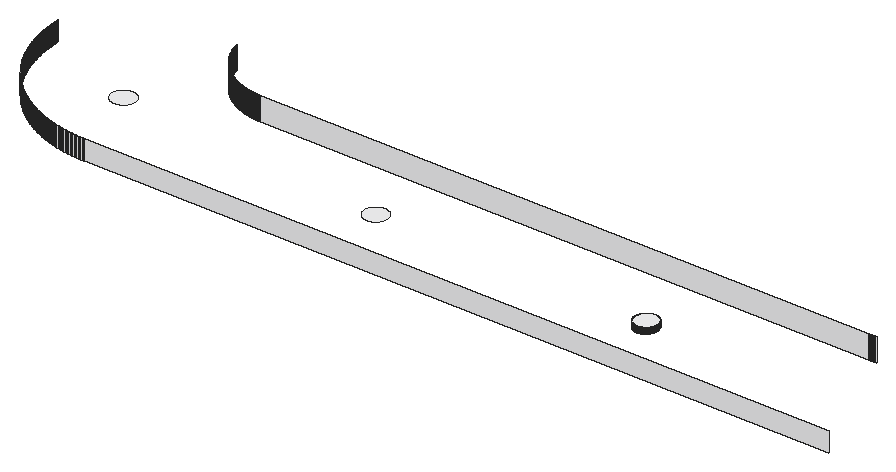
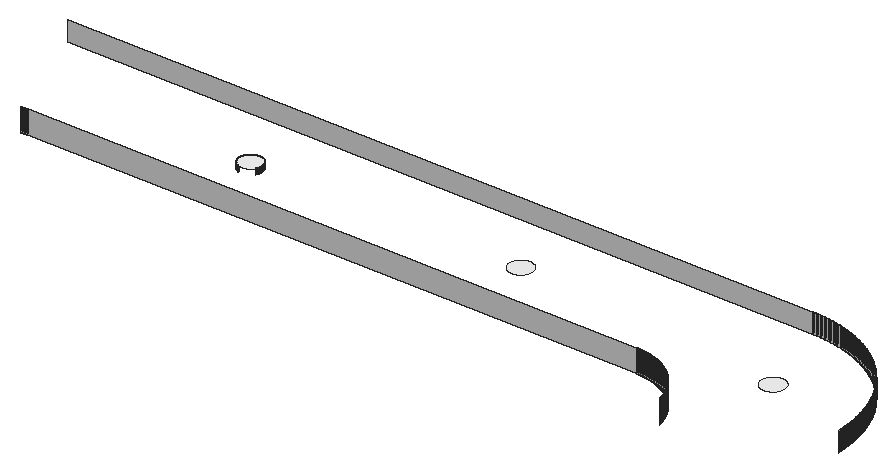
# SketchUp Ruby script. Lengths in inches.
U = 1.inch
M = Sketchup.active_model
def pt(a) = Geom::Point3d.new(a.map { |v| v * U })
def face(e, loops, mat)
  f = e.add_face(loops[0].map { |a| pt(a) })
  loops[1..].each { |l| e.add_face(l.map { |a| pt(a) }).erase! }
  f.material = f.back_material = mat if mat
  f
end
# faces: each face lists its corners as indices into pts; further lists are holes
def faces(e, pts, list, mat = nil) = list.each { |f| face(e, (f[0].is_a?(Array) ? f : [f]).map { |l| l.map { |i| pts[i] } }, mat) }
# xy, xz, yz: faces in a plane at the given z, y or x. An outline is a flat list of corners, or four numbers for a rectangle; further outlines are holes
def ring(l) = l.size == 4 ? [[l[0], l[1]], [l[2], l[1]], [l[2], l[3]], [l[0], l[3]]] : l.each_slice(2).to_a
def flat(e, list, mat, &to3) = list.each { |f| face(e, (f[0].is_a?(Array) ? f : [f]).map { |l| ring(l).map { |u, v| to3.(u, v) } }, mat) }
def xy(e, z, list, mat = nil) = flat(e, list, mat) { |x, y| [x, y, z] }
def xz(e, y, list, mat = nil) = flat(e, list, mat) { |x, z| [x, y, z] }
def yz(e, x, list, mat = nil) = flat(e, list, mat) { |y, z| [x, y, z] }
def lines(e, pts, list) = list.each { |a, b| e.add_line(pt(pts[a]), pt(pts[b])) }
# prism: a flat outline (further loops are holes) pulled along v
def prism(e, loops, v, mat = nil)
  f = face(e, loops, mat); d = Geom::Vector3d.new(v.map { |x| x * U })
  f.pushpull(f.normal.samedirection?(d) ? d.length : -d.length)
end
def box(e, o, s, mat = nil) = prism(e, [[o, [o[0] + s[0], o[1], o[2]], [o[0] + s[0], o[1] + s[1], o[2]], [o[0], o[1] + s[1], o[2]]]], [0, 0, s[2]], mat)
def at(x, y, z, deg = 0) = Geom::Transformation.translation(pt([x, y, z])) * Geom::Transformation.rotation(ORIGIN, Z_AXIS, deg.degrees)
def axes(o, x, y, z) = Geom::Transformation.new([*x, 0, *y, 0, *z, 0, *pt(o).to_a, 1])
def part(name) = M.definitions.add(name)
# library, detail: a bought-in or finely detailed component or shape, given as its bounding box
def library(name, o, s) = part(name).tap { |d| box(d.entities, o, s) }
def detail(e, o, s) = box(e.add_group.entities, o, s)
def put(e, d, t, mat = nil) = e.add_instance(d, t).tap { |i| i.material = mat if mat }
def group(e, t, mat = nil) = e.add_group.tap { |g| g.transformation = t; g.material = mat if mat }.entities
root = M.entities
M.materials.add("[Quartz Light Grey]").color = [251, 251, 252]
xy(root,112.81,[[87.021,52,86.896,52.003,86.771,52.013,86.646,52.032,86.523,52.058,86.402,52.091,86.284,52.133,86.168,52.181,86.055,52.237,85.947,52.3,85.842,52.369,85.742,52.445,85.647,52.527,85.557,52.615,85.473,52.709,85.395,52.807,85.323,52.91,85.258,53.018,85.2,53.129,85.148,53.244,85.105,53.362,85.068,53.482,85.04,53.604,85.019,53.728,85.005,53.853,85,53.979,85.003,54.104,85.013,54.229,85.032,54.354,85.058,54.477,85.091,54.598,85.133,54.716,85.181,54.832,85.237,54.945,85.3,55.053,85.369,55.158,85.445,55.258,85.527,55.353,85.615,55.443,85.709,55.527,85.807,55.605,85.91,55.677,86.018,55.742,86.129,55.8,86.244,55.852,86.362,55.895,86.482,55.932,86.604,55.96,86.728,55.981,86.853,55.995,86.979,56,87.104,55.997,87.229,55.987,87.354,55.968,87.477,55.942,87.598,55.909,87.716,55.867,87.832,55.819,87.945,55.763,88.053,55.7,88.158,55.631,88.258,55.555,88.353,55.473,88.443,55.385,88.527,55.291,88.605,55.193,88.677,55.09,88.742,54.982,88.8,54.871,88.852,54.756,88.895,54.638,88.932,54.518,88.96,54.396,88.981,54.272,88.995,54.147,89,54.021,88.997,53.896,88.987,53.771,88.968,53.646,88.942,53.523,88.909,53.402,88.867,53.284,88.819,53.168,88.763,53.055,88.7,52.947,88.631,52.842,88.555,52.742,88.473,52.647,88.385,52.557,88.291,52.473,88.193,52.395,88.09,52.323,87.982,52.258,87.871,52.2,87.756,52.148,87.638,52.105,87.518,52.068,87.396,52.04,87.272,52.019,87.147,52.005],[135.021,52,134.896,52.003,134.771,52.013,134.646,52.032,134.523,52.058,134.402,52.091,134.284,52.133,134.168,52.181,134.055,52.237,133.947,52.3,133.842,52.369,133.742,52.445,133.647,52.527,133.557,52.615,133.473,52.709,133.395,52.807,133.323,52.91,133.258,53.018,133.2,53.129,133.148,53.244,133.105,53.362,133.068,53.482,133.04,53.604,133.019,53.728,133.005,53.853,133,53.979,133.003,54.104,133.013,54.229,133.032,54.354,133.058,54.477,133.091,54.598,133.133,54.716,133.181,54.832,133.237,54.945,133.3,55.053,133.369,55.158,133.445,55.258,133.527,55.353,133.615,55.443,133.709,55.527,133.807,55.605,133.91,55.677,134.018,55.742,134.129,55.8,134.244,55.852,134.362,55.895,134.482,55.932,134.604,55.96,134.728,55.981,134.853,55.995,134.979,56,135.104,55.997,135.229,55.987,135.354,55.968,135.477,55.942,135.598,55.909,135.716,55.867,135.832,55.819,135.945,55.763,136.053,55.7,136.158,55.631,136.258,55.555,136.353,55.473,136.443,55.385,136.527,55.291,136.605,55.193,136.677,55.09,136.742,54.982,136.8,54.871,136.852,54.756,136.895,54.638,136.932,54.518,136.96,54.396,136.981,54.272,136.995,54.147,137,54.021,136.997,53.896,136.987,53.771,136.968,53.646,136.942,53.523,136.909,53.402,136.867,53.284,136.819,53.168,136.763,53.055,136.7,52.947,136.631,52.842,136.555,52.742,136.473,52.647,136.385,52.557,136.291,52.473,136.193,52.395,136.09,52.323,135.982,52.258,135.871,52.2,135.756,52.148,135.638,52.105,135.518,52.068,135.396,52.04,135.272,52.019,135.147,52.005],[39.021,56,38.896,56.003,38.771,56.013,38.646,56.032,38.523,56.058,38.402,56.091,38.284,56.133,38.168,56.181,38.055,56.237,37.947,56.3,37.842,56.369,37.742,56.445,37.647,56.527,37.557,56.615,37.473,56.709,37.395,56.807,37.323,56.91,37.258,57.018,37.2,57.129,37.148,57.244,37.105,57.362,37.068,57.482,37.04,57.604,37.019,57.728,37.005,57.853,37,57.979,37.003,58.104,37.013,58.229,37.032,58.354,37.058,58.477,37.091,58.598,37.133,58.716,37.181,58.832,37.237,58.945,37.3,59.053,37.369,59.158,37.445,59.258,37.527,59.353,37.615,59.443,37.709,59.527,37.807,59.605,37.91,59.677,38.018,59.742,38.129,59.8,38.244,59.852,38.362,59.895,38.482,59.932,38.604,59.96,38.728,59.981,38.853,59.995,38.979,60,39.104,59.997,39.229,59.987,39.354,59.968,39.477,59.942,39.598,59.909,39.716,59.867,39.832,59.819,39.945,59.763,40.053,59.7,40.158,59.631,40.258,59.555,40.353,59.473,40.443,59.385,40.527,59.291,40.605,59.193,40.677,59.09,40.742,58.982,40.8,58.871,40.852,58.756,40.895,58.638,40.932,58.518,40.96,58.396,40.981,58.272,40.995,58.147,41,58.021,40.997,57.896,40.987,57.771,40.968,57.646,40.942,57.523,40.909,57.402,40.867,57.284,40.819,57.168,40.763,57.055,40.7,56.947,40.631,56.842,40.555,56.742,40.473,56.647,40.385,56.557,40.291,56.473,40.193,56.395,40.09,56.323,39.982,56.258,39.871,56.2,39.756,56.148,39.638,56.105,39.518,56.068,39.396,56.04,39.272,56.019,39.147,56.005]],"[Quartz Light Grey]")
xz(root,42,[[45,111.81,177,115.32]],"[Quartz Light Grey]")
xz(root,66,[[57,111.81,165,115.905]],"[Quartz Light Grey]")
p = [[43.242,42.064,111.81],[43.493,42.047,111.81],[43.493,42.047,115.32],[43.242,42.064,115.32],[43.744,42.033,111.81],[43.744,42.033,115.32],
  [43.995,42.021,111.81],[43.995,42.021,115.32],[44.246,42.012,111.81],[44.246,42.012,115.32],[44.497,42.005,111.81],[44.497,42.005,115.32],
  [44.749,42.001,111.81],[44.749,42.001,115.32],[45,42,111.81],[45,42,115.32],[42.242,42.159,111.81],[42.491,42.131,111.81],
  [42.491,42.131,115.32],[42.242,42.159,115.32],[42.741,42.107,111.81],[42.741,42.107,115.32],[42.992,42.084,111.81],[42.992,42.084,115.32],
  [41.494,42.257,111.81],[41.743,42.222,111.81],[41.743,42.222,115.32],[41.494,42.257,115.32],[41.992,42.189,111.81],[41.992,42.189,115.32],
  [40.75,42.379,111.81],[40.998,42.336,111.81],[40.998,42.336,115.32],[40.75,42.379,115.32],[41.246,42.295,111.81],[41.246,42.295,115.32],
  [40.256,42.473,111.81],[40.503,42.425,111.81],[40.503,42.425,115.32],[40.256,42.473,115.32],[39.765,42.578,111.81],[40.01,42.524,111.81],
  [40.01,42.524,115.32],[39.765,42.578,115.32],[39.275,42.693,111.81],[39.52,42.634,111.81],[39.52,42.634,115.32],[39.275,42.693,115.32],
  [39.031,42.754,111.81],[39.031,42.754,115.32],[38.546,42.884,111.81],[38.788,42.818,111.81],[38.788,42.818,115.32],[38.546,42.884,115.32],
  [38.304,42.953,111.81],[38.304,42.953,115.32],[37.823,43.098,111.81],[38.063,43.024,111.81],[38.063,43.024,115.32],[37.823,43.098,115.32],
  [37.584,43.175,111.81],[37.584,43.175,115.32],[37.345,43.254,111.81],[37.345,43.254,115.32],[36.87,43.419,111.81],[37.107,43.335,111.81],
  [37.107,43.335,115.32],[36.87,43.419,115.32],[36.634,43.505,111.81],[36.634,43.505,115.32],[36.399,43.594,111.81],[36.399,43.594,115.32],
  [36.165,43.685,111.81],[36.165,43.685,115.32],[35.932,43.779,111.81],[35.932,43.779,115.32],[35.7,43.875,111.81],[35.7,43.875,115.32],
  [35.468,43.974,111.81],[35.468,43.974,115.32],[35.238,44.075,111.81],[35.238,44.075,115.32],[35.009,44.178,111.81],[35.009,44.178,115.32],
  [34.781,44.284,111.81],[34.781,44.284,115.32],[34.554,44.392,111.81],[34.554,44.392,115.32],[34.329,44.503,111.81],[34.329,44.503,115.32],
  [34.104,44.616,111.81],[34.104,44.616,115.32],[33.881,44.731,111.81],[33.881,44.731,115.32],[33.659,44.849,111.81],[33.659,44.849,115.32],
  [33.438,44.969,111.81],[33.438,44.969,115.32],[33.218,45.091,111.81],[33.218,45.091,115.32],[33,45.215,111.81],[33,45.215,115.32],
  [32.783,45.342,111.81],[32.783,45.342,115.32],[32.567,45.471,111.81],[32.567,45.471,115.32],[32.353,45.603,111.81],[32.353,45.603,115.32],
  [32.14,45.736,111.81],[32.14,45.736,115.32],[31.929,45.872,111.81],[31.929,45.872,115.32],[31.719,46.01,111.81],[31.719,46.01,115.32],
  [31.51,46.15,111.81],[31.51,46.15,115.32],[31.303,46.292,111.81],[31.303,46.292,115.32],[31.097,46.437,111.81],[31.097,46.437,115.32],
  [30.893,46.584,111.81],[30.893,46.584,115.32],[30.691,46.732,111.81],[30.691,46.732,115.32],[30.49,46.883,111.81],[30.49,46.883,115.32],
  [30.29,47.036,111.81],[30.29,47.036,115.32],[30.092,47.191,111.81],[30.092,47.191,115.32],[29.896,47.348,111.81],[29.896,47.348,115.32],
  [29.702,47.508,111.81],[29.702,47.508,115.32],[29.509,47.669,111.81],[29.509,47.669,115.32],[29.318,47.832,111.81],[29.318,47.832,115.32],
  [29.129,47.997,111.81],[29.129,47.997,115.32],[28.941,48.165,111.81],[28.941,48.165,115.32],[28.755,48.334,111.81],[28.755,48.334,115.32],
  [28.571,48.505,111.81],[28.571,48.505,115.32],[28.389,48.678,111.81],[28.389,48.678,115.32],[28.208,48.853,111.81],[28.208,48.853,115.32],
  [28.029,49.029,111.81],[28.029,49.029,115.32],[27.853,49.208,111.81],[27.853,49.208,115.32],[27.678,49.389,111.81],[27.678,49.389,115.32],
  [27.505,49.571,111.81],[27.505,49.571,115.32],[27.334,49.755,111.81],[27.334,49.755,115.32],[27.165,49.941,111.81],[27.165,49.941,115.32],
  [26.997,50.129,111.81],[26.997,50.129,115.32],[26.832,50.318,111.81],[26.832,50.318,115.32],[26.669,50.509,111.81],[26.669,50.509,115.32],
  [26.508,50.702,111.81],[26.508,50.702,115.32],[26.348,50.896,111.81],[26.348,50.896,115.32],[26.191,51.092,111.81],[26.191,51.092,115.32],
  [26.036,51.29,111.81],[26.036,51.29,115.32],[25.883,51.49,111.81],[25.883,51.49,115.32],[25.732,51.691,111.81],[25.732,51.691,115.32],
  [25.584,51.893,111.81],[25.584,51.893,115.32],[25.437,52.097,111.81],[25.437,52.097,115.32],[134.646,52.032,111.81],[134.523,52.058,111.81],
  [134.523,52.058,112.81],[134.646,52.032,112.81],[134.771,52.013,111.81],[134.771,52.013,112.81],[134.896,52.003,111.81],[134.896,52.003,112.81],
  [135.021,52,111.81],[135.021,52,112.81],[135.147,52.005,111.81],[135.147,52.005,112.81],[135.272,52.019,111.81],[135.272,52.019,112.81],
  [135.396,52.04,111.81],[135.396,52.04,112.81],[135.518,52.068,111.81],[135.518,52.068,112.81],[25.292,52.303,111.81],[25.292,52.303,115.32],
  [134.284,52.133,111.81],[134.168,52.181,111.81],[134.168,52.181,112.81],[134.284,52.133,112.81],[134.402,52.091,111.81],[134.402,52.091,112.81],
  [135.638,52.105,111.81],[135.638,52.105,112.81],[135.756,52.148,111.81],[135.756,52.148,112.81],[135.871,52.2,111.81],[135.871,52.2,112.81],
  [134.055,52.237,111.81],[133.947,52.3,111.81],[133.947,52.3,112.81],[134.055,52.237,112.81],[135.982,52.258,111.81],[135.982,52.258,112.81],
  [25.15,52.51,111.81],[25.15,52.51,115.32],[133.842,52.369,111.81],[133.842,52.369,112.81],[136.09,52.323,111.81],[136.09,52.323,112.81],
  [136.193,52.395,111.81],[136.193,52.395,112.81],[133.742,52.445,111.81],[133.647,52.527,111.81],[133.647,52.527,112.81],[133.742,52.445,112.81],
  [136.291,52.473,111.81],[136.291,52.473,112.81],[25.01,52.719,111.81],[25.01,52.719,115.32],[133.557,52.615,111.81],[133.557,52.615,112.81],
  [136.385,52.557,111.81],[136.385,52.557,112.81],[133.473,52.709,111.81],[133.473,52.709,112.81],[136.473,52.647,111.81],[136.473,52.647,112.81],
  [136.555,52.742,111.81],[136.555,52.742,112.81],[24.872,52.929,111.81],[24.872,52.929,115.32],[133.395,52.807,111.81],[133.395,52.807,112.81],
  [136.631,52.842,111.81],[136.631,52.842,112.81],[133.323,52.91,111.81],[133.323,52.91,112.81],[136.7,52.947,111.81],[136.7,52.947,112.81],
  [24.736,53.14,111.81],[24.736,53.14,115.32],[133.258,53.018,111.81],[133.258,53.018,112.81],[136.763,53.055,111.81],[136.763,53.055,112.81],
  [133.2,53.129,111.81],[133.2,53.129,112.81],[24.603,53.353,111.81],[24.603,53.353,115.32],[133.148,53.244,111.81],[133.148,53.244,112.81],
  [136.819,53.168,111.81],[136.819,53.168,112.81],[133.105,53.362,111.81],[133.105,53.362,112.81],[136.867,53.284,111.81],[136.867,53.284,112.81],
  [136.909,53.402,111.81],[136.909,53.402,112.81],[24.471,53.567,111.81],[24.471,53.567,115.32],[133.068,53.482,111.81],[133.068,53.482,112.81],
  [136.942,53.523,111.81],[136.942,53.523,112.81],[133.04,53.604,111.81],[133.04,53.604,112.81],[136.968,53.646,111.81],[136.968,53.646,112.81],
  [24.342,53.783,111.81],[24.342,53.783,115.32],[133.019,53.728,111.81],[133.019,53.728,112.81],[136.987,53.771,111.81],[136.987,53.771,112.81],
  [133.005,53.853,111.81],[133.005,53.853,112.81],[24.215,54,111.81],[24.215,54,115.32],[136.997,53.896,111.81],[136.997,53.896,112.81],
  [133,53.979,111.81],[133,53.979,112.81],[137,54.021,111.81],[137,54.021,112.81],[24.091,54.218,111.81],[24.091,54.218,115.32],
  [133.003,54.104,111.81],[133.003,54.104,112.81],[136.995,54.147,111.81],[136.995,54.147,112.81],[133.013,54.229,111.81],[133.013,54.229,112.81],
  [136.981,54.272,111.81],[136.981,54.272,112.81],[23.969,54.438,111.81],[23.969,54.438,115.32],[133.032,54.354,111.81],[133.032,54.354,112.81],
  [136.96,54.396,111.81],[136.96,54.396,112.81],[23.849,54.659,111.81],[23.849,54.659,115.32],[133.058,54.477,111.81],[133.058,54.477,112.81],
  [136.932,54.518,111.81],[136.932,54.518,112.81],[133.091,54.598,111.81],[133.091,54.598,112.81],[136.895,54.638,111.81],[136.895,54.638,112.81],
  [133.133,54.716,111.81],[133.133,54.716,112.81],[136.852,54.756,111.81],[136.852,54.756,112.81],[23.731,54.881,111.81],[23.731,54.881,115.32],
  [133.181,54.832,111.81],[133.181,54.832,112.81],[133.237,54.945,111.81],[133.237,54.945,112.81],[136.8,54.871,111.81],[136.8,54.871,112.81],
  [23.616,55.104,111.81],[23.616,55.104,115.32],[133.3,55.053,111.81],[133.3,55.053,112.81],[136.742,54.982,111.81],[136.742,54.982,112.81],
  [136.677,55.09,111.81],[136.677,55.09,112.81],[23.503,55.329,111.81],[23.503,55.329,115.32],[136.605,55.193,111.81],[136.605,55.193,112.81],
  [136.527,55.291,111.81],[136.527,55.291,112.81],[23.392,55.554,111.81],[23.392,55.554,115.32],[136.443,55.385,111.81],[136.443,55.385,112.81],
  [136.353,55.473,111.81],[136.353,55.473,112.81],[136.258,55.555,111.81],[136.258,55.555,112.81],[23.284,55.781,111.81],[23.284,55.781,115.32],
  [136.053,55.7,111.81],[136.158,55.631,111.81],[136.158,55.631,112.81],[136.053,55.7,112.81],[135.945,55.763,111.81],[135.945,55.763,112.81],
  [23.178,56.009,111.81],[23.178,56.009,115.32],[135.716,55.867,111.81],[135.832,55.819,111.81],[135.832,55.819,112.81],[135.716,55.867,112.81],
  [135.477,55.942,111.81],[135.598,55.909,111.81],[135.598,55.909,112.81],[135.477,55.942,112.81],[23.075,56.238,111.81],[23.075,56.238,115.32],
  [22.974,56.468,111.81],[22.974,56.468,115.32],[22.875,56.7,111.81],[22.875,56.7,115.32],[22.779,56.932,111.81],[22.779,56.932,115.32],
  [22.685,57.165,111.81],[22.685,57.165,115.32],[22.594,57.399,111.81],[22.594,57.399,115.32],[22.505,57.634,111.81],[22.505,57.634,115.32],
  [22.419,57.87,111.81],[22.419,57.87,115.32],[22.335,58.107,111.81],[22.335,58.107,115.32],[22.254,58.345,111.81],[22.254,58.345,115.32],
  [22.175,58.584,111.81],[22.175,58.584,115.32],[22.098,58.823,111.81],[22.098,58.823,115.32],[22.024,59.063,111.81],[22.024,59.063,115.32],
  [21.953,59.304,111.81],[21.953,59.304,115.32],[21.884,59.546,111.81],[21.884,59.546,115.32],[21.818,59.788,111.81],[21.818,59.788,115.32],
  [21.754,60.031,111.81],[21.754,60.031,115.32],[21.693,60.275,111.81],[21.693,60.275,115.32],[21.634,60.52,111.81],[21.634,60.52,115.32],
  [21.578,60.765,111.81],[21.578,60.765,115.32],[21.524,61.01,111.81],[21.524,61.01,115.32],[21.473,61.256,111.81],[21.473,61.256,115.32],
  [21.425,61.503,111.81],[21.425,61.503,115.32],[21.379,61.75,111.81],[21.379,61.75,115.32],[21.336,61.998,111.81],[21.336,61.998,115.32],
  [21.295,62.246,111.81],[21.295,62.246,115.32],[21.257,62.494,111.81],[21.257,62.494,115.32],[21.222,62.743,111.81],[21.222,62.743,115.32],
  [21.189,62.992,111.81],[21.189,62.992,115.32],[21.159,63.242,111.81],[21.159,63.242,115.32],[21.131,63.491,111.81],[21.131,63.491,115.32],
  [21.107,63.741,111.81],[21.107,63.741,115.32],[21.084,63.992,111.81],[21.084,63.992,115.32],[21.064,64.242,111.81],[21.064,64.242,115.32],
  [21.047,64.493,111.81],[21.047,64.493,115.32],[21.033,64.744,111.81],[21.033,64.744,115.32],[21.021,64.995,111.81],[21.021,64.995,115.32],
  [21.012,65.246,111.81],[21.012,65.246,115.32],[21.005,65.497,111.81],[21.005,65.497,115.32],[21.001,65.749,111.81],[21.001,65.749,115.32],
  [21,66,111.81],[21,66,115.32],[56.055,66.037,111.81],[55.898,66.051,111.81],[55.898,66.051,115.905],[56.055,66.037,115.905],
  [56.213,66.026,111.81],[56.213,66.026,115.905],[56.37,66.017,111.81],[56.37,66.017,115.905],[56.527,66.009,111.81],[56.527,66.009,115.905],
  [56.685,66.004,111.81],[56.685,66.004,115.905],[56.842,66.001,111.81],[56.842,66.001,115.905],[57,66,111.81],[57,66,115.905],
  [165.157,66.001,111.81],[165,66,111.81],[165,66,115.905],[165.157,66.001,115.905],[165.314,66.004,111.81],[165.314,66.004,115.905],
  [165.471,66.009,111.81],[165.471,66.009,115.905],[165.628,66.016,111.81],[165.628,66.016,115.905],[165.785,66.026,111.81],[165.785,66.026,115.905],
  [165.942,66.037,111.81],[165.942,66.037,115.905],[166.098,66.05,111.81],[166.098,66.05,115.905],[55.117,66.149,111.81],[54.961,66.174,111.81],
  [54.961,66.174,115.905],[55.117,66.149,115.905],[55.272,66.125,111.81],[55.272,66.125,115.905],[55.428,66.103,111.81],[55.428,66.103,115.905],
  [55.585,66.084,111.81],[55.585,66.084,115.905],[55.741,66.066,111.81],[55.741,66.066,115.905],[166.254,66.066,111.81],[166.254,66.066,115.905],
  [54.651,66.232,111.81],[54.497,66.264,111.81],[54.497,66.264,115.905],[54.651,66.232,115.905],[54.806,66.202,111.81],[54.806,66.202,115.905],
  [54.189,66.334,111.81],[54.037,66.372,111.81],[54.037,66.372,115.905],[54.189,66.334,115.905],[54.343,66.298,111.81],[54.343,66.298,115.905],
  [53.884,66.412,111.81],[53.732,66.454,111.81],[53.732,66.454,115.905],[53.884,66.412,115.905],[53.43,66.543,111.81],[53.28,66.591,111.81],
  [53.28,66.591,115.905],[53.43,66.543,115.905],[53.581,66.497,111.81],[53.581,66.497,115.905],[53.13,66.641,111.81],[52.981,66.693,111.81],
  [52.981,66.693,115.905],[53.13,66.641,115.905],[52.833,66.747,111.81],[52.686,66.802,111.81],[52.686,66.802,115.905],[52.833,66.747,115.905],
  [52.539,66.86,111.81],[52.539,66.86,115.905],[52.393,66.919,111.81],[52.248,66.981,111.81],[52.248,66.981,115.905],[52.393,66.919,115.905],
  [52.104,67.044,111.81],[51.96,67.11,111.81],[51.96,67.11,115.905],[52.104,67.044,115.905],[51.818,67.177,111.81],[51.818,67.177,115.905],
  [51.676,67.246,111.81],[51.535,67.316,111.81],[51.535,67.316,115.905],[51.676,67.246,115.905],[51.395,67.389,111.81],[51.395,67.389,115.905],
  [51.257,67.464,111.81],[51.257,67.464,115.905],[51.119,67.54,111.81],[50.982,67.618,111.81],[50.982,67.618,115.905],[51.119,67.54,115.905],
  [50.846,67.698,111.81],[50.846,67.698,115.905],[50.711,67.78,111.81],[50.711,67.78,115.905],[50.578,67.863,111.81],[50.578,67.863,115.905],
  [50.445,67.949,111.81],[50.314,68.035,111.81],[50.314,68.035,115.905],[50.445,67.949,115.905],[50.183,68.124,111.81],[50.183,68.124,115.905],
  [50.054,68.215,111.81],[50.054,68.215,115.905],[49.926,68.307,111.81],[49.926,68.307,115.905],[49.8,68.4,111.81],[49.8,68.4,115.905],
  [49.674,68.496,111.81],[49.674,68.496,115.905],[49.55,68.593,111.81],[49.55,68.593,115.905],[49.427,68.691,111.81],[49.427,68.691,115.905],
  [49.305,68.792,111.81],[49.305,68.792,115.905],[49.185,68.894,111.81],[49.185,68.894,115.905],[49.066,68.997,111.81],[49.066,68.997,115.905],
  [48.949,69.102,111.81],[48.949,69.102,115.905],[48.832,69.208,111.81],[48.832,69.208,115.905],[48.718,69.316,111.81],[48.718,69.316,115.905],
  [48.604,69.426,111.81],[48.604,69.426,115.905],[48.492,69.537,111.81],[48.492,69.537,115.905],[48.382,69.649,111.81],[48.382,69.649,115.905],
  [48.273,69.763,111.81],[48.273,69.763,115.905],[48.166,69.879,111.81],[48.166,69.879,115.905],[48.06,69.995,111.81],[48.06,69.995,115.905],
  [47.955,70.113,111.81],[47.955,70.113,115.905],[47.853,70.233,111.81],[47.853,70.233,115.905],[47.751,70.354,111.81],[47.751,70.354,115.905],
  [47.652,70.476,111.81],[47.652,70.476,115.905],[47.554,70.599,111.81],[47.554,70.599,115.905],[47.457,70.724,111.81],[47.457,70.724,115.905],
  [47.363,70.85,111.81],[47.363,70.85,115.905],[47.27,70.977,111.81],[47.27,70.977,115.905],[47.178,71.105,111.81],[47.178,71.105,115.905],
  [47.089,71.235,111.81],[47.089,71.235,115.905],[47.001,71.366,111.81],[47.001,71.366,115.905],[46.914,71.498,111.81],[46.914,71.498,115.905],
  [46.83,71.631,111.81],[46.83,71.631,115.905],[46.747,71.765,111.81],[46.747,71.765,115.905],[46.666,71.9,111.81],[46.666,71.9,115.905],
  [46.587,72.036,111.81],[46.587,72.036,115.905],[46.509,72.174,111.81],[46.509,72.174,115.905],[46.434,72.312,111.81],[46.434,72.312,115.905],
  [46.36,72.451,111.81],[46.36,72.451,115.905],[46.288,72.591,111.81],[46.288,72.591,115.905],[46.218,72.732,111.81],[46.218,72.732,115.905],
  [46.15,72.875,111.81],[46.15,72.875,115.905],[46.083,73.017,111.81],[46.083,73.017,115.905],[46.019,73.161,111.81],[46.019,73.161,115.905],
  [45.956,73.306,111.81],[45.956,73.306,115.905],[45.895,73.451,111.81],[45.895,73.451,115.905],[45.837,73.598,111.81],[45.837,73.598,115.905],
  [45.78,73.745,111.81],[45.78,73.745,115.905],[45.725,73.892,111.81],[45.725,73.892,115.905],[45.672,74.041,111.81],[45.672,74.041,115.905],
  [45.621,74.19,111.81],[45.621,74.19,115.905],[45.572,74.34,111.81],[45.572,74.34,115.905],[45.525,74.49,111.81],[45.525,74.49,115.905],
  [45.48,74.641,111.81],[45.48,74.641,115.905],[45.436,74.793,111.81],[45.436,74.793,115.905],[45.395,74.945,111.81],[45.395,74.945,115.905],
  [45.356,75.097,111.81],[45.356,75.097,115.905],[45.319,75.251,111.81],[45.319,75.251,115.905],[45.004,66,111.81],[45,66,111.81]]
faces(root,p,[[0,1,2,3],[1,4,5,2],[4,6,7,5],[6,8,9,7],[8,10,11,9],[10,12,13,11],[12,14,15,13],[16,17,18,19],
  [17,20,21,18],[20,22,23,21],[22,0,3,23],[24,25,26,27],[25,28,29,26],[28,16,19,29],[30,31,32,33],[31,34,35,32],
  [34,24,27,35],[36,37,38,39],[37,30,33,38],[40,41,42,43],[41,36,39,42],[44,45,46,47],[45,40,43,46],[48,44,47,49],
  [50,51,52,53],[51,48,49,52],[54,50,53,55],[56,57,58,59],[57,54,55,58],[60,56,59,61],[62,60,61,63],[64,65,66,67],
  [65,62,63,66],[68,64,67,69],[70,68,69,71],[72,70,71,73],[74,72,73,75],[76,74,75,77],[78,76,77,79],[80,78,79,81],
  [82,80,81,83],[84,82,83,85],[86,84,85,87],[88,86,87,89],[90,88,89,91],[92,90,91,93],[94,92,93,95],[96,94,95,97],
  [98,96,97,99],[100,98,99,101],[102,100,101,103],[104,102,103,105],[106,104,105,107],[108,106,107,109],[110,108,109,111],[112,110,111,113],
  [114,112,113,115],[116,114,115,117],[118,116,117,119],[120,118,119,121],[122,120,121,123],[124,122,123,125],[126,124,125,127],[128,126,127,129],
  [130,128,129,131],[132,130,131,133],[134,132,133,135],[136,134,135,137],[138,136,137,139],[140,138,139,141],[142,140,141,143],[144,142,143,145],
  [146,144,145,147],[148,146,147,149],[150,148,149,151],[152,150,151,153],[154,152,153,155],[156,154,155,157],[158,156,157,159],[160,158,159,161],
  [162,160,161,163],[164,162,163,165],[166,164,165,167],[168,166,167,169],[170,168,169,171],[172,170,171,173],[174,172,173,175],[176,174,175,177],
  [178,176,177,179],[180,178,179,181],[182,180,181,183],[184,185,186,187],[188,184,187,189],[190,188,189,191],[192,190,191,193],[194,192,193,195],
  [196,194,195,197],[198,196,197,199],[200,198,199,201],[202,182,183,203],[204,205,206,207],[208,204,207,209],[185,208,209,186],[210,200,201,211],
  [212,210,211,213],[214,212,213,215],[216,217,218,219],[205,216,219,206],[220,214,215,221],[222,202,203,223],[217,224,225,218],[226,220,221,227],
  [228,226,227,229],[230,231,232,233],[224,230,233,225],[234,228,229,235],[236,222,223,237],[231,238,239,232],[240,234,235,241],[238,242,243,239],
  [244,240,241,245],[246,244,245,247],[248,236,237,249],[242,250,251,243],[252,246,247,253],[250,254,255,251],[256,252,253,257],[258,248,249,259],
  [254,260,261,255],[262,256,257,263],[260,264,265,261],[266,258,259,267],[264,268,269,265],[270,262,263,271],[268,272,273,269],[274,270,271,275],
  [276,274,275,277],[278,266,267,279],[272,280,281,273],[282,276,277,283],[280,284,285,281],[286,282,283,287],[288,278,279,289],[284,290,291,285],
  [292,286,287,293],[290,294,295,291],[296,288,289,297],[298,292,293,299],[294,300,301,295],[302,298,299,303],[304,296,297,305],[300,306,307,301],
  [308,302,303,309],[306,310,311,307],[312,308,309,313],[314,304,305,315],[310,316,317,311],[318,312,313,319],[320,314,315,321],[316,322,323,317],
  [324,318,319,325],[322,326,327,323],[328,324,325,329],[326,330,331,327],[332,328,329,333],[334,320,321,335],[330,336,337,331],[336,338,339,337],
  [340,332,333,341],[342,334,335,343],[338,344,345,339],[346,340,341,347],[348,346,347,349],[350,342,343,351],[352,348,349,353],[354,352,353,355],
  [356,350,351,357],[358,354,355,359],[360,358,359,361],[362,360,361,363],[364,356,357,365],[366,367,368,369],[367,362,363,368],[370,366,369,371],
  [372,364,365,373],[374,375,376,377],[375,370,371,376],[378,379,380,381],[379,374,377,380],[382,372,373,383],[384,382,383,385],[386,384,385,387],
  [388,386,387,389],[390,388,389,391],[392,390,391,393],[394,392,393,395],[396,394,395,397],[398,396,397,399],[400,398,399,401],[402,400,401,403],
  [404,402,403,405],[406,404,405,407],[408,406,407,409],[410,408,409,411],[412,410,411,413],[414,412,413,415],[416,414,415,417],[418,416,417,419],
  [420,418,419,421],[422,420,421,423],[424,422,423,425],[426,424,425,427],[428,426,427,429],[430,428,429,431],[432,430,431,433],[434,432,433,435],
  [436,434,435,437],[438,436,437,439],[440,438,439,441],[442,440,441,443],[444,442,443,445],[446,444,445,447],[448,446,447,449],[450,448,449,451],
  [452,450,451,453],[454,452,453,455],[456,454,455,457],[458,456,457,459],[460,458,459,461],[462,460,461,463],[464,465,466,467],[468,464,467,469],
  [470,468,469,471],[472,470,471,473],[474,472,473,475],[476,474,475,477],[478,476,477,479],[480,481,482,483],[484,480,483,485],[486,484,485,487],
  [488,486,487,489],[490,488,489,491],[492,490,491,493],[494,492,493,495],[496,497,498,499],[500,496,499,501],[502,500,501,503],[504,502,503,505],
  [506,504,505,507],[465,506,507,466],[508,494,495,509],[510,511,512,513],[514,510,513,515],[497,514,515,498],[516,517,518,519],[520,516,519,521],
  [511,520,521,512],[522,523,524,525],[517,522,525,518],[526,527,528,529],[530,526,529,531],[523,530,531,524],[532,533,534,535],[527,532,535,528],
  [536,537,538,539],[533,536,539,534],[537,540,541,538],[542,543,544,545],[540,542,545,541],[546,547,548,549],[543,546,549,544],[547,550,551,548],
  [552,553,554,555],[550,552,555,551],[553,556,557,554],[556,558,559,557],[560,561,562,563],[558,560,563,559],[561,564,565,562],[564,566,567,565],
  [566,568,569,567],[570,571,572,573],[568,570,573,569],[571,574,575,572],[574,576,577,575],[576,578,579,577],[578,580,581,579],[580,582,583,581],
  [582,584,585,583],[584,586,587,585],[586,588,589,587],[588,590,591,589],[590,592,593,591],[592,594,595,593],[594,596,597,595],[596,598,599,597],
  [598,600,601,599],[600,602,603,601],[602,604,605,603],[604,606,607,605],[606,608,609,607],[608,610,611,609],[610,612,613,611],[612,614,615,613],
  [614,616,617,615],[616,618,619,617],[618,620,621,619],[620,622,623,621],[622,624,625,623],[624,626,627,625],[626,628,629,627],[628,630,631,629],
  [630,632,633,631],[632,634,635,633],[634,636,637,635],[636,638,639,637],[638,640,641,639],[640,642,643,641],[642,644,645,643],[644,646,647,645],
  [646,648,649,647],[648,650,651,649],[650,652,653,651],[652,654,655,653],[654,656,657,655],[656,658,659,657],[658,660,661,659],[660,662,663,661],
  [662,664,665,663],[664,666,667,665],[666,668,669,667],[668,670,671,669],[670,672,673,671],[672,674,675,673],[674,676,677,675],[676,678,679,677],
  [678,680,681,679],[680,682,683,681],[682,684,685,683],[684,686,687,685]],"[Quartz Light Grey]")
lines(root,p,[[688,689]])
